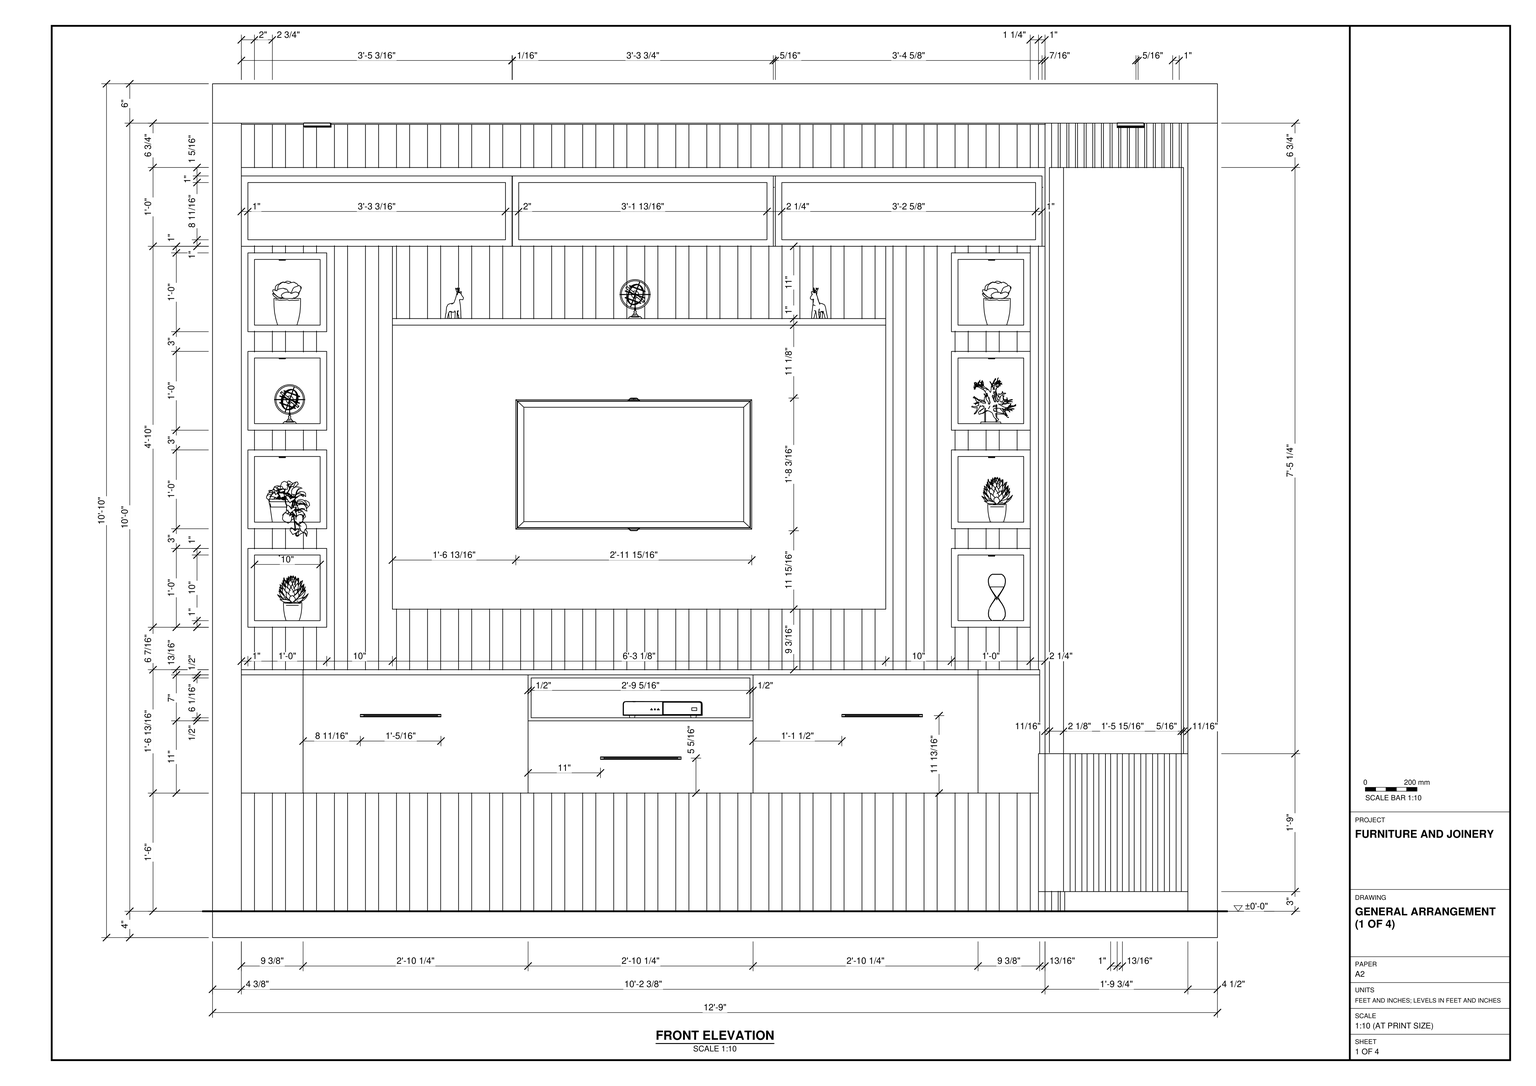
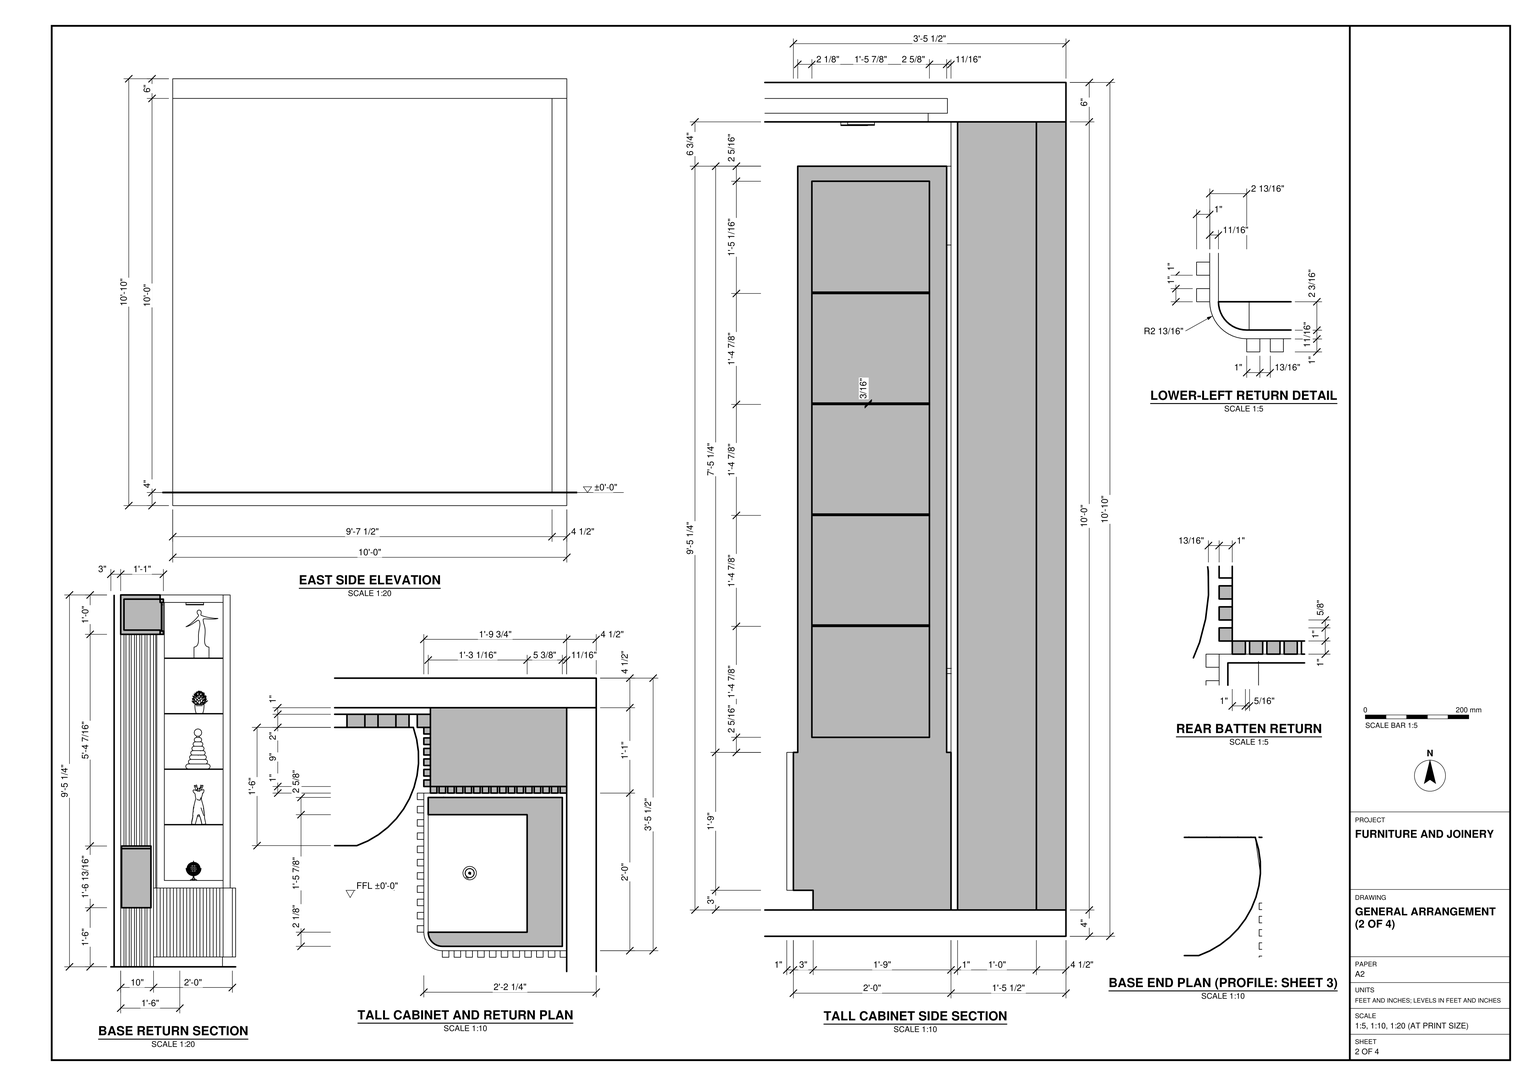
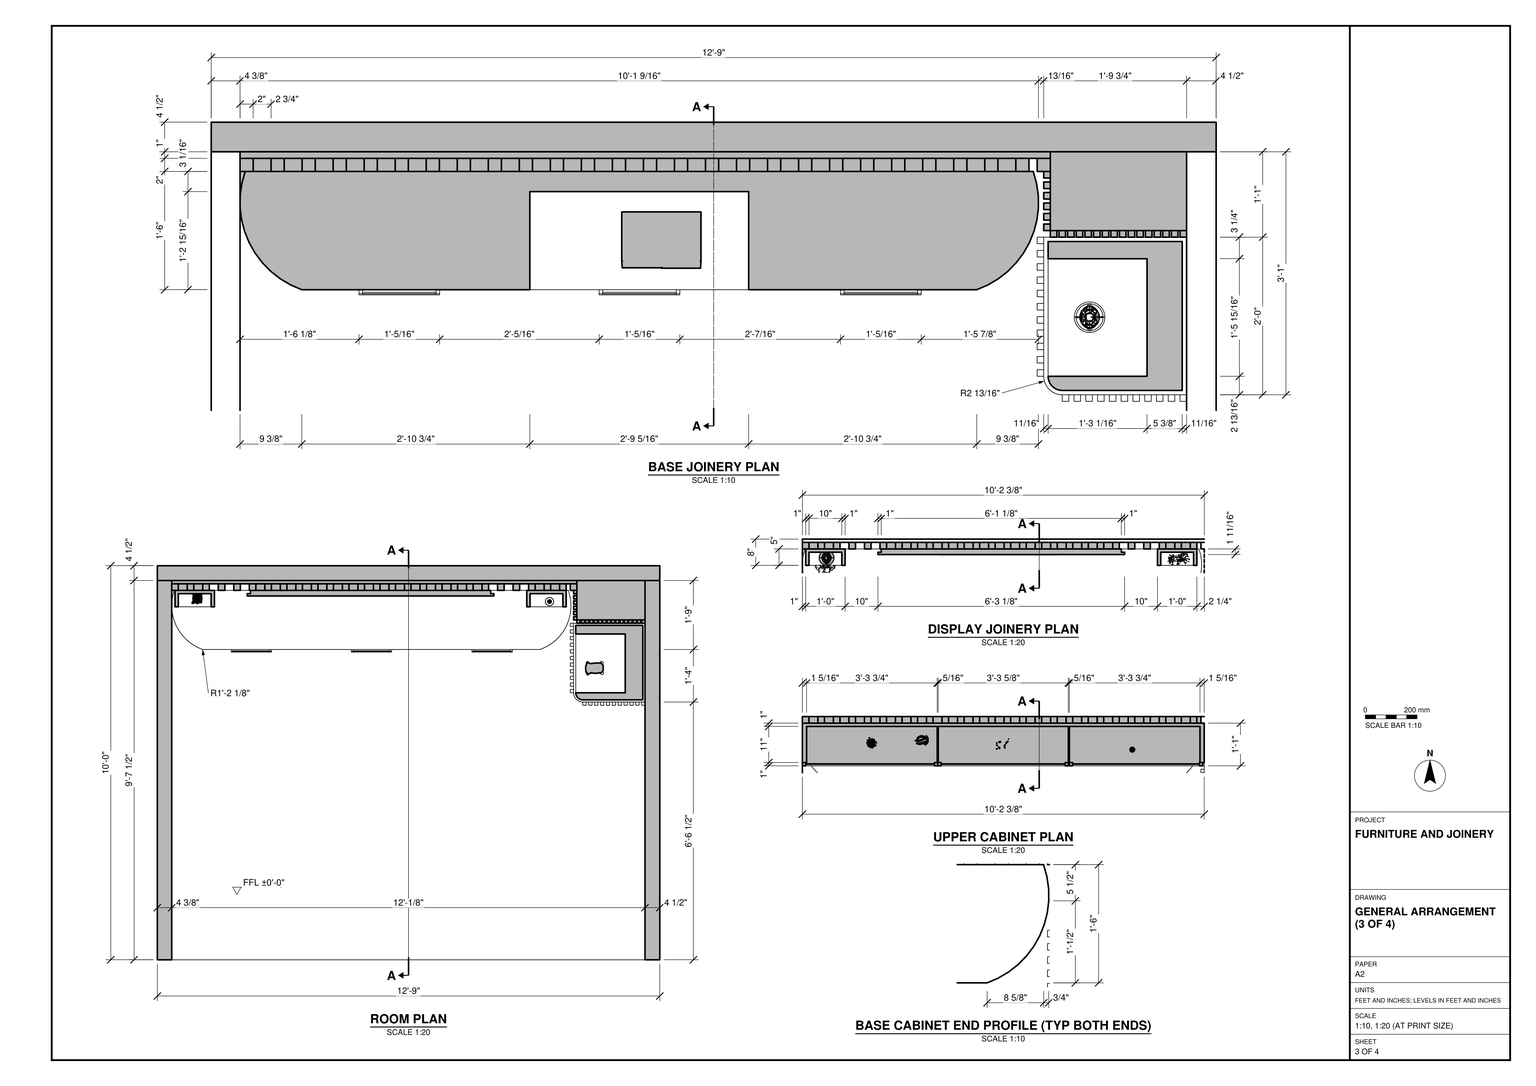
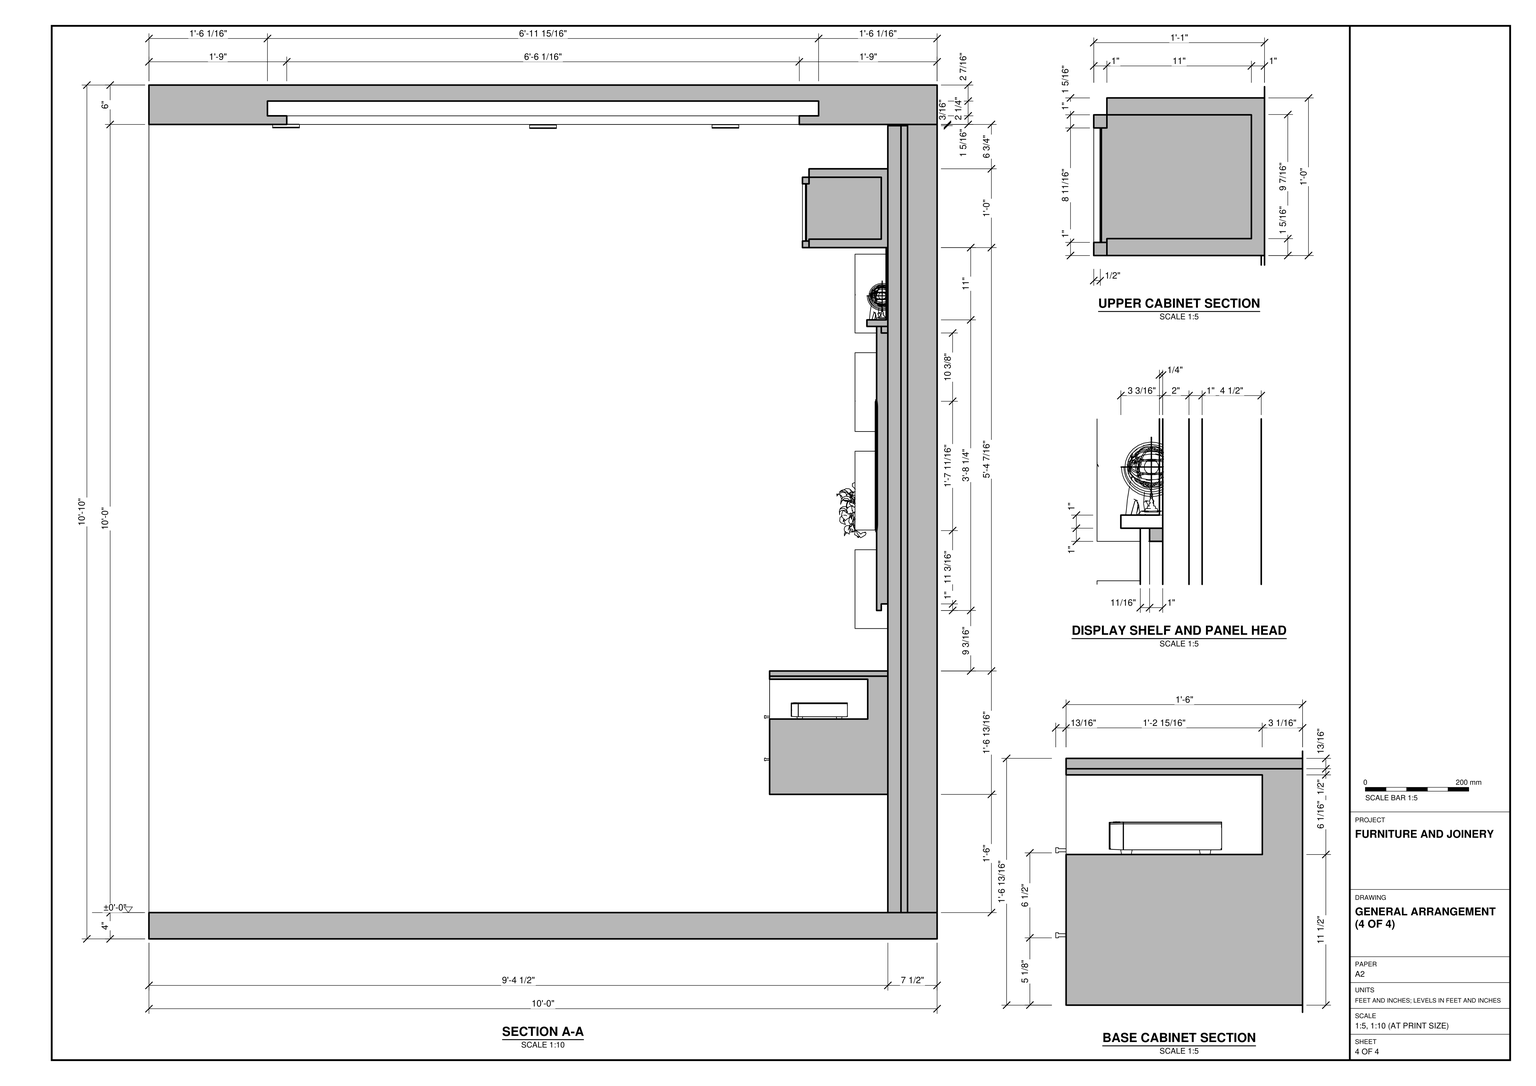
Use task_files/diagram_01.pdf to model the television wall and its room shell in SketchUp. Work in feet and inches. The overall model is 12'-9" wide, 10'-0" deep and 10'-10" high, with the finished floor at ±0'-0". Build the floor slab, ceiling slab, rear wall and two side walls to the thicknesses shown in the plans and sections. Leave the front open as drawn.

Use the front elevation to set out the vertical battens, the central television panel and its display ledge. Flank the panel with matching stacks of square display boxes and span the main display with a row of three upper cabinet bays. Below the television, model the raised base cabinet with horizontal pulls and an open equipment compartment above the middle drawer. Use the plan and end profile to shape both curved ends of the cabinet. At the right, turn the joinery out from the wall to form the tall cabinet, with its display shelves facing sideways and its rounded, battened base return. Place the television, media equipment, plants and display objects in the locations shown. Decor and loose items may be any suitable library components, for example from 3D Warehouse.

Keep shell elements and individual furniture or joinery pieces in separate groups or components, and use components for repeated parts. Save one SketchUp model as output_files/built_in_television_wall_with_a_side_display_cabinet.skp.

# SketchUp Ruby script. Lengths in inches.
U = 1.inch
M = Sketchup.active_model
def pt(a) = Geom::Point3d.new(a.map { |v| v * U })
def face(e, loops, mat)
  f = e.add_face(loops[0].map { |a| pt(a) })
  loops[1..].each { |l| e.add_face(l.map { |a| pt(a) }).erase! }
  f.material = f.back_material = mat if mat
  f
end
# faces: each face lists its corners as indices into pts; further lists are holes
def faces(e, pts, list, mat = nil) = list.each { |f| face(e, (f[0].is_a?(Array) ? f : [f]).map { |l| l.map { |i| pts[i] } }, mat) }
# xy, xz, yz: faces in a plane at the given z, y or x. An outline is a flat list of corners, or four numbers for a rectangle; further outlines are holes
def ring(l) = l.size == 4 ? [[l[0], l[1]], [l[2], l[1]], [l[2], l[3]], [l[0], l[3]]] : l.each_slice(2).to_a
def flat(e, list, mat, &to3) = list.each { |f| face(e, (f[0].is_a?(Array) ? f : [f]).map { |l| ring(l).map { |u, v| to3.(u, v) } }, mat) }
def xy(e, z, list, mat = nil) = flat(e, list, mat) { |x, y| [x, y, z] }
def xz(e, y, list, mat = nil) = flat(e, list, mat) { |x, z| [x, y, z] }
def yz(e, x, list, mat = nil) = flat(e, list, mat) { |y, z| [x, y, z] }
def lines(e, pts, list) = list.each { |a, b| e.add_line(pt(pts[a]), pt(pts[b])) }
# prism: a flat outline (further loops are holes) pulled along v
def prism(e, loops, v, mat = nil)
  f = face(e, loops, mat); d = Geom::Vector3d.new(v.map { |x| x * U })
  f.pushpull(f.normal.samedirection?(d) ? d.length : -d.length)
end
def box(e, o, s, mat = nil) = prism(e, [[o, [o[0] + s[0], o[1], o[2]], [o[0] + s[0], o[1] + s[1], o[2]], [o[0], o[1] + s[1], o[2]]]], [0, 0, s[2]], mat)
def at(x, y, z, deg = 0) = Geom::Transformation.translation(pt([x, y, z])) * Geom::Transformation.rotation(ORIGIN, Z_AXIS, deg.degrees)
def axes(o, x, y, z) = Geom::Transformation.new([*x, 0, *y, 0, *z, 0, *pt(o).to_a, 1])
def part(name) = M.definitions.add(name)
# library, detail: a bought-in or finely detailed component or shape, given as its bounding box
def library(name, o, s) = part(name).tap { |d| box(d.entities, o, s) }
def detail(e, o, s) = box(e.add_group.entities, o, s)
def put(e, d, t, mat = nil) = e.add_instance(d, t).tap { |i| i.material = mat if mat }
def group(e, t, mat = nil) = e.add_group.tap { |g| g.transformation = t; g.material = mat if mat }.entities
root = M.entities
M.materials.add("Carpaint Black Matte 1.5cm").color = [255, 255, 255]
M.materials.add("Emissive").color = [255, 201, 138]
M.materials.add("Emissive\#1").color = [255, 201, 138]
M.materials.add("Marble Beige 23-58 150cm").color = [206, 178, 147]
M.materials.add("Marble Black 01 150cm").color = [31, 31, 31]
M.materials.add("Marble White 602 38.29cm").color = [255, 255, 255]
M.materials.add("Tiles Marble White 03 180cm").color = [241, 241, 241]
M.materials.add("Wood Teak 33-35 100cm").color = [135, 81, 33]
M.materials.add("XPS Yellow SSS 1.51cm").color = [255, 255, 255]
M.materials.add("glass").color = [129, 129, 129]
M.materials["glass"].alpha = 0.1
c1 = part("Vertical slat \#1")
xy(c1.entities,0,[[-1,0,0,1]])
xy(c1.entities,21,[[-1,0,0,1]],"Wood Teak 33-35 100cm")
xz(c1.entities,0,[[-1,0,0,21]],"Wood Teak 33-35 100cm")
xz(c1.entities,1,[[-1,0,0,21]])
yz(c1.entities,-1,[[0,0,1,21]],"Wood Teak 33-35 100cm")
yz(c1.entities,0,[[0,0,1,21]])
c2 = part("Vertical slat")
xy(c2.entities,0,[[0,-1,1,0]])
xy(c2.entities,21,[[0,-1,1,0]],"Wood Teak 33-35 100cm")
xz(c2.entities,-1,[[0,0,1,21]],"Wood Teak 33-35 100cm")
xz(c2.entities,0,[[0,0,1,21]])
yz(c2.entities,0,[[-1,0,0,21]],"Wood Teak 33-35 100cm")
yz(c2.entities,1,[[-1,0,0,21]],"Wood Teak 33-35 100cm")
c3 = library("Tlon Light 650 Ceiling 152 007",[-12.8,-12.8,-3.78],[25.6,25.6,3.58])
c4 = library("Spot Light",[-5.1,-5.1,-11.05],[10.2,10.2,11.05])
c5 = library("Potted Plant 50-23",[-3.4,-3.5,0],[6.8,7,9.93])
c6 = library("Potted Plant 50-24",[-2.18,-2.1,0],[4.36,4.2,6.7])
c7 = library("Decorative Deer 209 004",[-1.58,-4.16,0],[3.36,7.25,10.63])
c8 = library("Plant 260 031 02",[-5.66,-10.61,-5.67],[17.04,23.05,21.91])
c9 = library("Sculpture 108-23",[-12.84,-6.01,0],[25.68,12.02,38.36])
c10 = library("Tree Decoration 83-10",[-18.61,-13.07,0],[43.1,29.04,44.77])
c11 = library("Armillary Sphere 37-31",[-7.11,-7.1,0],[14.21,14.18,18.13])
c12 = library("Toy Wooden Pyramid 40-01",[-3.18,-3.18,0],[6.36,6.36,10.41])
c13 = library("Decorative Hourglass 001",[-1.06,-1.06,0.02],[2.12,2.12,5.71])
c14 = part("OuterShell")
prism(c14.entities,[[[0,0,0.08],[0,0,0.31],[0,0.59,0.31],[0,0.59,0.39],[0,0.79,0.39],[0,0.79,0],[0,0.59,0],[0,0.59,0.08]]],[0.39,0,0])
c15 = part("Cabinet pull")
put(c15.entities,c14,at(0,0,0))
put(c15.entities,c14,at(8.62,0,0))
g1 = group(c15.entities,at(0,0,0))
g2 = group(g1,at(0,0,0.2))
xy(g2,0,[[0.39,0.39,8.62,0.79]])
xy(g2,0.12,[[0.39,0.39,8.62,0.59]])
xy(g2,0.2,[[0.39,0.59,8.62,0.63],[0.39,0.63,8.62,0.79]])
xz(g2,0.39,[[0.39,0,8.62,0.12]])
xz(g2,0.59,[[0.39,0.12,8.62,0.2]])
xz(g2,0.79,[[0.39,0,8.62,0.2]])
yz(g2,0.39,[[0.39,0,0.39,0.12,0.59,0.12,0.59,0.2,0.79,0.2,0.79,0]])
yz(g2,8.62,[[0.39,0,0.79,0,0.79,0.2,0.59,0.2,0.59,0.12,0.39,0.12]])
g3 = group(g1,at(0,0,0.2))
xy(g3,-0.2,[[0.39,0.59,8.62,0.63],[0.39,0.63,8.62,0.79]])
xy(g3,-0.12,[[0.39,0.39,8.62,0.59]])
xy(g3,0,[[0.39,0.39,8.62,0.79]])
xz(g3,0.39,[[0.39,-0.12,8.62,0]])
xz(g3,0.59,[[0.39,-0.2,8.62,-0.12]])
xz(g3,0.79,[[0.39,-0.2,8.62,0]])
yz(g3,0.39,[[0.59,-0.2,0.79,-0.2,0.79,0,0.39,0,0.39,-0.12,0.59,-0.12]])
yz(g3,8.62,[[0.59,-0.2,0.59,-0.12,0.39,-0.12,0.39,0,0.79,0,0.79,-0.2]])
c16 = library("Flat screen television",[0,1.41,1.14],[35.92,0.28,20.21])
c17 = library("skpE36B",[-3.84,-2.73,0],[7.68,5.46,1.59])
c18 = part("Vertical wall slat \#1")
box(c18.entities,[0,-1,0],[1,1,120])
c19 = part("Vertical wall slat \#2")
box(c19.entities,[-1,0,0],[1,1,120])
c20 = part("Vertical wall slat")
box(c20.entities,[0,-2,0],[2,2,119.8125])
c21 = part("Group\#7")
xy(c21.entities,0,[[0,0,12,5]])
xy(c21.entities,1,[[1,0,11,4]])
xy(c21.entities,11,[[1,0,11,4]])
xy(c21.entities,12,[[0,0,12,5]])
xz(c21.entities,0,[[[0,0,12,12],[1,1,11,11]]])
xz(c21.entities,4,[[1,1,11,11]])
xz(c21.entities,5,[[0,0,12,12]])
yz(c21.entities,0,[[0,0,5,12]])
yz(c21.entities,1,[[0,1,4,11]])
yz(c21.entities,11,[[0,1,4,11]])
yz(c21.entities,12,[[0,0,5,12]])
c22 = library("Group\#18",[0,0,0],[122.36,13,12])
xy(root,4,[[0,0,4.39,115.5]])
xy(root,124,[[0,0,4.39,115.5],[[4.39,0,4.39,115.5,0,115.5,0,120,153,120,153,0],[25.37,20.98,131.02,99.02]]])
xy(root,125.3125,[[22.43,18.04,134.96,18.04,134.96,101.96,131.89,101.96,131.89,99.02,131.02,99.02,131.02,20.98,25.37,20.98,25.37,99.02,131.89,99.02,131.89,101.96,22.43,101.96]],"Emissive\#1")
xy(root,127.5625,[[22.43,18.04,134.96,101.96]])
xy(root,130,[[0,0,153,120]])
xz(root,0,[[0,4,4.39,124],[0,124,153,130]])
xz(root,18.04,[[22.43,125.3125,134.96,127.5625]])
xz(root,20.98,[[25.37,124,131.02,125.3125]])
xz(root,99.02,[[25.37,124,131.02,125.3125]])
xz(root,101.96,[[22.43,125.3125,134.96,127.5625]])
xz(root,115.5,[[0,4,4.39,124]])
xz(root,120,[[0,124,153,130]])
yz(root,0,[[0,4,115.5,124],[0,124,120,130]])
yz(root,4.39,[[0,4,115.5,124]])
yz(root,22.43,[[18.04,125.3125,101.96,127.5625]])
yz(root,25.37,[[20.98,124,99.02,125.3125]])
yz(root,131.02,[[20.98,124,99.02,125.3125]])
yz(root,134.96,[[18.04,125.3125,101.96,127.5625]])
yz(root,153,[[0,124,120,130]])
put(root,c1,at(126.75,101.5,7))
put(root,c1,at(126.75,99.48,7))
put(root,c1,at(126.75,97.46,7))
put(root,c1,at(126.75,95.45,7))
put(root,c1,at(126.75,93.43,7))
put(root,c1,at(126.75,91.41,7))
put(root,c1,at(126.75,89.39,7))
put(root,c1,at(126.75,87.37,7))
put(root,c1,at(126.75,85.35,7))
put(root,c1,at(126.75,83.34,7))
put(root,c1,at(126.75,81.32,7))
put(root,c2,at(147.5,78.5,7))
put(root,c2,at(129.57,78.5,7))
put(root,c2,at(145.71,78.5,7))
put(root,c2,at(143.91,78.5,7))
put(root,c2,at(142.12,78.5,7))
put(root,c2,at(140.33,78.5,7))
put(root,c2,at(138.53,78.5,7))
put(root,c2,at(136.74,78.5,7))
put(root,c2,at(134.95,78.5,7))
put(root,c2,at(133.15,78.5,7))
put(root,c2,at(131.36,78.5,7))
put(root,c3,axes([133.1,89.95,115],[0.21,0,0],[0,0.21,0],[0,0,0.21]))
put(root,c4,axes([35.08,110.23,105.24],[0.4,0,0],[0,0.36,0],[0,0,0.34]))
put(root,c4,axes([96.25,110.23,105.24],[0.4,0,0],[0,0.36,0],[0,0,0.34]))
put(root,c4,axes([63.45,110.23,105.24],[0.4,0,0],[0,0.36,0],[0,0,0.34]))
put(root,c3,axes([10.62,109.9,103.26],[0.03744,0,0],[0,0.03744,0],[0,0,0.03744]))
put(root,c3,axes([10.62,109.9,88.26],[0.03744,0,0],[0,0.03744,0],[0,0,0.03744]))
put(root,c3,axes([10.62,109.9,73.2],[0.03744,0,0],[0,0.03744,0],[0,0,0.03744]))
put(root,c3,axes([10.62,109.9,58.2],[0.03744,0,0],[0,0.03744,0],[0,0,0.03744]))
put(root,c3,axes([118.62,109.9,58.2],[0.03744,0,0],[0,0.03744,0],[0,0,0.03744]))
put(root,c3,axes([118.62,109.9,73.2],[0.03744,0,0],[0,0.03744,0],[0,0,0.03744]))
put(root,c3,axes([118.62,109.9,88.26],[0.03744,0,0],[0,0.03744,0],[0,0,0.03744]))
put(root,c3,axes([118.62,109.9,103.26],[0.03744,0,0],[0,0.03744,0],[0,0,0.03744]))
put(root,c5,axes([12.23,109.91,48.25],[0.69,0,0],[0,0.69,0],[0,0,0.69]))
put(root,c6,at(11.33,109.6,93.25))
put(root,c7,axes([132.77,88.9,47.39],[0,-1.29,0],[1,0,0],[0,0,1.13]))
put(root,c8,axes([10.39,108.79,63.25],[0.38618,0,0],[0,0.38618,0],[0,0,0.38618]))
put(root,c9,axes([129.7,87.75,98.07],[0,-0.38,0],[0.38,0,0],[0,0,0.38]))
put(root,c10,axes([118.49,109.55,78.25],[0.15644,0,0],[0,0.15644,0],[0,0,0.15644]))
put(root,c11,axes([11.74,109.83,78.25],[0.3276,0,0],[0,0.3276,0],[0,0,0.3276]))
put(root,c12,axes([133.51,88.98,64.28],[0,-1.17,0],[1.17,0,0],[0,0,1.17]))
put(root,c13,axes([119.42,109.1,48.23],[1.24,0,0],[0,1.24,0],[0,0,1.24]))
put(root,c5,axes([119.46,109.91,63.25],[0.69,0,0],[0,0.69,0],[0,0,0.69]))
put(root,c6,at(119.39,109.6,93.25))
put(root,c5,axes([132.16,88.41,81.18],[0.69,0,0],[0,0.69,0],[0,0,0.69]))
put(root,c11,axes([133.73,90.32,30.3],[0.3276,0,0],[0,0.3276,0],[0,0,0.3276]))
put(root,c15,axes([22.5,94.5,33.99],[1.3624,0,0],[0,-1,0],[0,0,-1]))
put(root,c15,axes([95.8125,94.5,33.99],[1.3624,0,0],[0,-1,0],[0,0,-1]))
put(root,c15,axes([59.0625,94.5,27.52],[1.3624,0,0],[0,-1,0],[0,0,-1]))
put(root,c3,axes([15.9,20.87,124.08],[0.1596,0,0],[0,0.1596,0],[0,0,0.1596]))
put(root,c3,axes([139.76,20.98,124.08],[0.1596,0,0],[0,0.1596,0],[0,0,0.1596]))
put(root,c3,axes([139.76,88.8125,124.08],[0.1596,0,0],[0,0.1596,0],[0,0,0.1596]))
put(root,c3,axes([16.02,87.77,124.03],[0.1596,0,0],[0,0.1596,0],[0,0,0.1596]))
put(root,c3,axes([139.76,60,123.92],[0.1596,0,0],[0,0.1596,0],[0,0,0.1596]))
put(root,c3,axes([16.02,60,123.99],[0.1596,0,0],[0,0.1596,0],[0,0,0.1596]))
put(root,c7,axes([36.75,110.73,94.25],[0.25155,0.4357,0],[-0.33775,0.195,0],[0,0,0.4407]))
put(root,c7,axes([92.26,111.04,94.25],[0.32406,-0.38483,0],[0.29832,0.25121,0],[0,0,0.4407]))
put(root,c11,axes([64.34,111.64,94.25],[0.3276,0,0],[0,0.3276,0],[0,0,0.3276]))
put(root,c16,at(46.17,109.21,60.8))
put(root,c17,axes([68.53,102.06,33.47],[1.57,0,0],[0,1.57,0],[0,0,1.57]))
put(root,c5,axes([25.55,106.33,106.47],[0.69,0,0],[0,0.69,0],[0,0,0.69]))
put(root,c6,at(40.53,107.34,106.54))
put(root,c10,axes([65.76,106.09,106.54],[0.15644,0,0],[0,0.15644,0],[0,0,0.15644]))
put(root,c12,axes([104.85,104.44,106.54],[0,-0.7488,0],[0.7488,0,0],[0,0,0.7488]))
g4 = group(root,at(33,0,0))
box(g4,[-33,0,0],[153,120,4],"Tiles Marble White 03 180cm")
g5 = group(root,at(33,115.5,4))
xy(g5,0,[[-33,0,120,4.5]])
xy(g5,120,[[-33,0,120,4.5]])
xz(g5,0,[[-33,0,120,120]],"XPS Yellow SSS 1.51cm")
xz(g5,4.5,[[-33,0,120,120]])
yz(g5,-33,[[0,0,4.5,120]])
yz(g5,120,[[0,0,4.5,120]])
g6 = group(root,at(148.5,0,4))
xy(g6,0,[[0,0,4.5,115.5]])
xy(g6,120,[[0,0,4.5,115.5]])
xz(g6,0,[[0,0,4.5,120]])
xz(g6,115.5,[[0,0,4.5,120]])
yz(g6,0,[[0,0,115.5,120]],"XPS Yellow SSS 1.51cm")
yz(g6,4.5,[[0,0,115.5,120]])
g7 = group(root,at(5.17,94.5,22))
xy(g7,0,[[8.62,0,6.92,0.73,5.33,1.67,3.88,2.81,2.59,4.13,1.49,5.61,0.58,7.21,-0.11,8.93,-0.5625,10.72,-0.78,12.55,-0.76,14.4,-0.5,16.22,0,18,120,18,120,17.93,120.49,16.16,120.75,14.34,120.77,12.5,120.55,10.67,120.09,8.89,119.4,7.18,118.5,5.58,117.39,4.11,116.11,2.79,114.66,1.66,113.07,0.72,111.38,0]])
xy(g7,11.47,[[43.34,0,76.66,14.9375]],"Wood Teak 33-35 100cm")
xy(g7,17.53,[[43.34,0,76.66,14.9375]],"Wood Teak 33-35 100cm")
xy(g7,18,[[8.62,0,6.92,0.73,5.33,1.67,3.88,2.81,2.59,4.13,1.49,5.61,0.58,7.21,-0.11,8.93,-0.5625,10.72,-0.78,12.55,-0.76,14.4,-0.5,16.22,0,18,120,18,120,17.93,120.49,16.16,120.75,14.34,120.77,12.5,120.55,10.67,120.09,8.89,119.4,7.18,118.5,5.58,117.39,4.11,116.11,2.79,114.66,1.66,113.07,0.72,111.38,0]])
xy(g7,18.79,[[8.62,0,111.38,0,113.07,0.72,114.66,1.66,116.11,2.79,117.39,4.11,118.5,5.58,119.4,7.18,120.09,8.89,120.55,10.67,120.77,12.5,120.75,14.34,120.49,16.16,120,17.93,120,18,0,18,-0.5,16.22,-0.76,14.4,-0.78,12.55,-0.5625,10.72,-0.11,8.93,0.58,7.21,1.49,5.61,2.59,4.13,3.88,2.81,5.33,1.67,6.92,0.73]],"Marble Black 01 150cm")
xz(g7,0,[[8.62,18,111.38,18.79]],"Marble Black 01 150cm")
xz(g7,0,[[8.62,0,42.87,18],[42.87,0,77.13,11],[77.13,0,111.38,18]],"Marble White 602 38.29cm")
xz(g7,0,[[[42.87,11,77.13,18],[43.34,11.47,76.66,17.53]]],"Wood Teak 33-35 100cm")
xz(g7,14.9375,[[43.34,11.47,76.66,17.53]],"Wood Teak 33-35 100cm")
xz(g7,18,[[0,0,120,18],[0,18,120,18.79]])
yz(g7,43.34,[[0,11.47,14.9375,17.53]],"Wood Teak 33-35 100cm")
yz(g7,76.66,[[0,11.47,14.9375,17.53]],"Wood Teak 33-35 100cm")
yz(g7,120,[[17.93,0,18,18],[17.93,18,18,18.79]])
p = [[8.62,0,0],[8.62,0,18],[6.92,0.73,18],[6.92,0.73,0],[113.07,0.72,0],[113.07,0.72,18],
  [111.38,0,18],[111.38,0,0],[5.33,1.67,18],[5.33,1.67,0],[114.66,1.66,0],[114.66,1.66,18],
  [3.88,2.81,18],[3.88,2.81,0],[116.11,2.79,0],[116.11,2.79,18],[2.59,4.13,18],[2.59,4.13,0],
  [117.39,4.11,0],[117.39,4.11,18],[1.49,5.61,18],[1.49,5.61,0],[118.5,5.58,0],[118.5,5.58,18],
  [0.58,7.21,18],[0.58,7.21,0],[119.4,7.18,0],[119.4,7.18,18],[-0.11,8.93,18],[-0.11,8.93,0],
  [120.09,8.89,0],[120.09,8.89,18],[-0.5625,10.72,18],[-0.5625,10.72,0],[120.55,10.67,0],[120.55,10.67,18],
  [-0.78,12.55,18],[-0.78,12.55,0],[120.77,12.5,0],[120.77,12.5,18],[-0.76,14.4,18],[-0.76,14.4,0],
  [120.75,14.34,0],[120.75,14.34,18],[120.49,16.16,0],[120.49,16.16,18],[-0.5,16.22,18],[-0.5,16.22,0],
  [0,18,18],[0,18,0],[120,17.93,0],[120,17.93,18],[8.62,0,18.79],[6.92,0.73,18.79],
  [113.07,0.72,18.79],[111.38,0,18.79],[5.33,1.67,18.79],[114.66,1.66,18.79],[3.88,2.81,18.79],[116.11,2.79,18.79],
  [2.59,4.13,18.79],[117.39,4.11,18.79],[1.49,5.61,18.79],[118.5,5.58,18.79],[0.58,7.21,18.79],[119.4,7.18,18.79],
  [-0.11,8.93,18.79],[120.09,8.89,18.79],[-0.5625,10.72,18.79],[120.55,10.67,18.79],[-0.78,12.55,18.79],[120.77,12.5,18.79],
  [-0.76,14.4,18.79],[120.75,14.34,18.79],[120.49,16.16,18.79],[-0.5,16.22,18.79],[0,18,18.79],[120,17.93,18.79]]
faces(g7,p,[[0,1,2,3],[4,5,6,7],[3,2,8,9],[10,11,5,4],[9,8,12,13],[14,15,11,10],[13,12,16,17],[18,19,15,14],
  [17,16,20,21],[22,23,19,18],[21,20,24,25],[26,27,23,22],[24,28,29,25],[26,30,31,27],[28,32,33,29],[30,34,35,31],
  [32,36,37,33],[34,38,39,35],[36,40,41,37],[38,42,43,39],[42,44,45,43],[40,46,47,41],[46,48,49,47],[44,50,51,45]],"Marble White 602 38.29cm")
faces(g7,p,[[2,1,52,53],[6,5,54,55],[8,2,53,56],[5,11,57,54],[12,8,56,58],[11,15,59,57],[16,12,58,60],[15,19,61,59],
  [20,16,60,62],[19,23,63,61],[24,20,62,64],[23,27,65,63],[28,24,64,66],[27,31,67,65],[32,28,66,68],[31,35,69,67],
  [36,32,68,70],[35,39,71,69],[40,36,70,72],[39,43,73,71],[43,45,74,73],[46,40,72,75],[48,46,75,76],[45,51,77,74]],"Marble Black 01 150cm")
g8 = group(root,at(124.5,103.5,4),"Wood Teak 33-35 100cm")
xy(g8,0,[[3.25,0,24,12]])
xy(g8,120,[[3.25,0,24,12]])
xz(g8,0,[[4.25,0,24,120]])
xz(g8,12,[[3.25,0,24,120]])
yz(g8,3.25,[[1,0,12,120]])
yz(g8,24,[[0,0,12,120]])
put(g8,c18,at(3.25,0,0))
put(g8,c18,at(4.57,0,0))
put(g8,c18,at(5.88,0,0))
put(g8,c18,at(7.2,0,0))
put(g8,c18,at(8.52,0,0))
put(g8,c18,at(9.83,0,0))
put(g8,c18,at(11.15,0,0))
put(g8,c18,at(12.47,0,0))
put(g8,c18,at(13.78,0,0))
put(g8,c18,at(15.1,0,0))
put(g8,c18,at(16.42,0,0))
put(g8,c18,at(17.73,0,0))
put(g8,c18,at(19.05,0,0))
put(g8,c18,at(20.37,0,0))
put(g8,c18,at(21.68,0,0))
put(g8,c18,at(23,0,0))
put(g8,c19,at(3.25,0,0))
put(g8,c19,at(3.25,1.6,0))
put(g8,c19,at(3.25,3.2,0))
put(g8,c19,at(3.25,4.8,0))
put(g8,c19,at(3.25,6.4,0))
put(g8,c19,at(3.25,8,0))
g9 = group(root,at(4.39,114.5,4),"Wood Teak 33-35 100cm")
xy(g9,0,[[0,0,123.36,1]])
xy(g9,119.8125,[[0,0,123.36,1]])
xz(g9,0,[[2,0,123.36,119.8125]])
xz(g9,1,[[0,0,123.36,119.8125]])
yz(g9,0,[[0,0,1,119.8125]])
yz(g9,123.36,[[0,0,1,119.8125]])
put(g9,c20,at(0,0,0))
put(g9,c20,at(4.72,0,0))
put(g9,c20,at(9.45,0,0))
put(g9,c20,at(14.17,0,0))
put(g9,c20,at(18.9,0,0))
put(g9,c20,at(23.62,0,0))
put(g9,c20,at(28.35,0,0))
put(g9,c20,at(33.07,0,0))
put(g9,c20,at(37.8,0,0))
put(g9,c20,at(42.52,0,0))
put(g9,c20,at(47.25,0,0))
put(g9,c20,at(51.97,0,0))
put(g9,c20,at(56.69,0,0))
put(g9,c20,at(61.42,0,0))
put(g9,c20,at(66.14,0,0))
put(g9,c20,at(70.87,0,0))
put(g9,c20,at(75.59,0,0))
put(g9,c20,at(80.32,0,0))
put(g9,c20,at(85.04,0,0))
put(g9,c20,at(89.77,0,0))
put(g9,c20,at(94.49,0,0))
put(g9,c20,at(99.22,0,0))
put(g9,c20,at(103.94,0,0))
put(g9,c20,at(108.66,0,0))
put(g9,c20,at(113.39,0,0))
put(g9,c20,at(118.11,0,0))
put(g9,c20,at(121.36,0,0))
g10 = group(root,at(27.39,110.79,50))
xy(g10,0,[[0,0,75.11,0.71]])
xy(g10,1,[[1,0.71,74.11,1.71]],"Emissive")
xy(g10,42.25,[[1,0.71,74.11,1.71]],"Emissive")
xy(g10,43.25,[[0,0,75.11,0.71]])
xz(g10,0,[[0,0,75.11,43.25]],"Marble Beige 23-58 150cm")
xz(g10,0.71,[[[0,0,75.11,43.25],[1,1,74.11,42.25]]])
xz(g10,1.71,[[1,1,74.11,42.25]])
yz(g10,0,[[0,0,0.71,43.25]])
yz(g10,1,[[0.71,1,1.71,42.25]],"Emissive")
yz(g10,74.11,[[0.71,1,1.71,42.25]],"Emissive")
yz(g10,75.11,[[0,0,0.71,43.25]])
g11 = group(root,at(5.39,107.5,47.25),"Marble White 602 38.29cm")
put(g11,c21,at(0,0,30))
put(g11,c21,at(107.11,0,30))
put(g11,c21,at(107.11,0,0))
put(g11,c21,at(107.11,0,15))
put(g11,c21,at(0,0,15))
put(g11,c21,at(0,0,45))
put(g11,c21,at(107.11,0,45))
put(g11,c21,at(0,0,0))
put(root,c22,at(4.39,99.5,105.25),"Marble White 602 38.29cm")
g12 = group(root,at(126.75,78.5,4),"Marble White 602 38.29cm")
xy(g12,0,[[3,3,21.75,24]])
xy(g12,3,[[2.82,0,2.45,0.02,2.09,0.1,1.74,0.21,1.41,0.38,1.1,0.58,0.83,0.83,0.58,1.1,0.38,1.41,0.21,1.74,0.1,2.09,0.02,2.45,0,2.82,0,24,3,24,3,0],[3,0,21.75,3]])
xy(g12,24,[[[2.82,0,21.75,0,21.75,24,0,24,0,2.82,0.02,2.45,0.1,2.09,0.21,1.74,0.38,1.41,0.58,1.1,0.83,0.83,1.1,0.58,1.41,0.38,1.74,0.21,2.09,0.1,2.45,0.02],[2.82,0.67,2.54,0.68,2.26,0.74,1.99,0.83,1.74,0.95,1.51,1.11,1.3,1.3,1.11,1.51,0.95,1.74,0.83,1.99,0.74,2.26,0.68,2.54,0.67,2.82,0.67,23.33,21.08,23.33,21.08,0.67]]])
xy(g12,26.29,[[0.67,2.82,15.73,20.71]])
xy(g12,26.3,[[0.67,2.82,15.73,20.71]])
xy(g12,110.96,[[0.67,2.82,15.73,20.71]])
xy(g12,113.25,[[2.82,0.67,21.08,0.67,21.08,23.33,0.67,23.33,0.67,2.82,0.68,2.54,0.74,2.26,0.83,1.99,0.95,1.74,1.11,1.51,1.3,1.3,1.51,1.11,1.74,0.95,1.99,0.83,2.26,0.74,2.54,0.68]])
xz(g12,0,[[2.82,3,20.75,24]],"Wood Teak 33-35 100cm")
xz(g12,0.67,[[2.82,24,20.75,113.25],[20.75,24,21.08,113.25]])
xz(g12,2.82,[[0.67,26.29,15.73,26.3],[0.67,26.3,15.73,110.96]])
xz(g12,3,[[3,0,21.75,3]],"Wood Teak 33-35 100cm")
xz(g12,20.71,[[0.67,26.29,15.73,26.3],[0.67,26.3,15.73,110.96]])
xz(g12,23.33,[[0.67,24,21.08,113.25]])
xz(g12,24,[[3,0,3,3,0,3,0,24,21.75,24,21.75,0]])
yz(g12,0,[[2.82,3,23,24]],"Wood Teak 33-35 100cm")
yz(g12,0.67,[[2.82,24,2.82,26.29,20.71,26.29,20.71,110.96,2.82,110.96,2.82,113.25,23,113.25,23,24],[23,24,23.33,113.25],[2.82,26.29,20.71,26.3]])
yz(g12,3,[[3,0,24,3]],"Wood Teak 33-35 100cm")
yz(g12,15.73,[[2.82,26.29,20.71,26.3]])
yz(g12,15.73,[[2.82,26.3,20.71,110.96]],"Wood Teak 33-35 100cm")
yz(g12,21.08,[[0.67,24,23.33,113.25]])
yz(g12,21.75,[[3,0,24,0,24,24,0,24,0,3,3,3]])
p = [[2.45,0.02,24],[2.09,0.1,24],[2.09,0.1,3],[2.45,0.02,3],[2.82,0,24],[2.82,0,3],
  [1.74,0.21,24],[1.74,0.21,3],[1.41,0.38,24],[1.41,0.38,3],[1.1,0.58,24],[1.1,0.58,3],
  [0.83,0.83,24],[0.83,0.83,3],[0.58,1.1,24],[0.58,1.1,3],[0.38,1.41,24],[0.38,1.41,3],
  [0.21,1.74,24],[0.21,1.74,3],[0.1,2.09,24],[0.1,2.09,3],[0.02,2.45,24],[0.02,2.45,3],
  [0,2.82,24],[0,2.82,3],[1.99,0.83,24],[2.26,0.74,24],[2.26,0.74,113.25],[1.99,0.83,113.25],
  [2.54,0.68,24],[2.54,0.68,113.25],[2.82,0.67,24],[2.82,0.67,113.25],[1.74,0.95,24],[1.74,0.95,113.25],
  [1.51,1.11,24],[1.51,1.11,113.25],[1.3,1.3,24],[1.3,1.3,113.25],[1.11,1.51,24],[1.11,1.51,113.25],
  [0.95,1.74,24],[0.95,1.74,113.25],[0.83,1.99,24],[0.83,1.99,113.25],[0.74,2.26,24],[0.74,2.26,113.25],
  [0.68,2.54,24],[0.68,2.54,113.25],[0.67,2.82,24],[0.67,2.82,113.25],[0.67,2.82,110.96],[0.67,2.82,26.3],
  [0.67,2.82,26.29]]
faces(g12,p,[[0,1,2,3],[4,0,3,5],[1,6,7,2],[6,8,9,7],[8,10,11,9],[10,12,13,11],[12,14,15,13],[14,16,17,15],
  [16,18,19,17],[18,20,21,19],[20,22,23,21],[22,24,25,23]],"Wood Teak 33-35 100cm")
faces(g12,p,[[26,27,28,29],[27,30,31,28],[30,32,33,31],[34,26,29,35],[36,34,35,37],[38,36,37,39],[40,38,39,41],[42,40,41,43],
  [44,42,43,45],[46,44,45,47],[48,46,47,49],[50,48,49,51,52,53,54]])
g13 = group(root,at(127.42,81.32,47.19))
xy(g13,0,[[0,0,15.0625,17.9]],"glass")
xy(g13,0.2,[[0,0,15.0625,17.9]],"glass")
xz(g13,0,[[0,0,15.0625,0.2]])
xz(g13,17.9,[[0,0,15.0625,0.2]])
yz(g13,0,[[0,0,17.9,0.2]],"glass")
yz(g13,15.0625,[[0,0,17.9,0.2]])
g14 = group(root,at(127.42,81.32,64.08))
xy(g14,0,[[0,0,15.0625,17.9]],"glass")
xy(g14,0.2,[[0,0,15.0625,17.9]],"glass")
xz(g14,0,[[0,0,15.0625,0.2]])
xz(g14,17.9,[[0,0,15.0625,0.2]])
yz(g14,0,[[0,0,17.9,0.2]],"glass")
yz(g14,15.0625,[[0,0,17.9,0.2]])
g15 = group(root,at(127.42,81.32,80.98))
xy(g15,0,[[0,0,15.0625,17.9]],"glass")
xy(g15,0.2,[[0,0,15.0625,17.9]],"glass")
xz(g15,0,[[0,0,15.0625,0.2]])
xz(g15,17.9,[[0,0,15.0625,0.2]])
yz(g15,0,[[0,0,17.9,0.2]],"glass")
yz(g15,15.0625,[[0,0,17.9,0.2]])
g16 = group(root,at(127.42,81.32,97.87))
xy(g16,0,[[0,0,15.0625,17.9]],"glass")
xy(g16,0.2,[[0,0,15.0625,17.9]],"glass")
xz(g16,0,[[0,0,15.0625,0.2]])
xz(g16,17.9,[[0,0,15.0625,0.2]])
yz(g16,0,[[0,0,17.9,0.2]],"glass")
yz(g16,15.0625,[[0,0,17.9,0.2]])
g17 = group(root,at(27.39,112.25,93.25),"Carpaint Black Matte 1.5cm")
prism(g17,[[[0,0.25,12],[0,0.25,0],[0,-2.9375,0],[0,-2.9375,1],[0,0,1],[0,0,12]]],[75.11,0,0])
